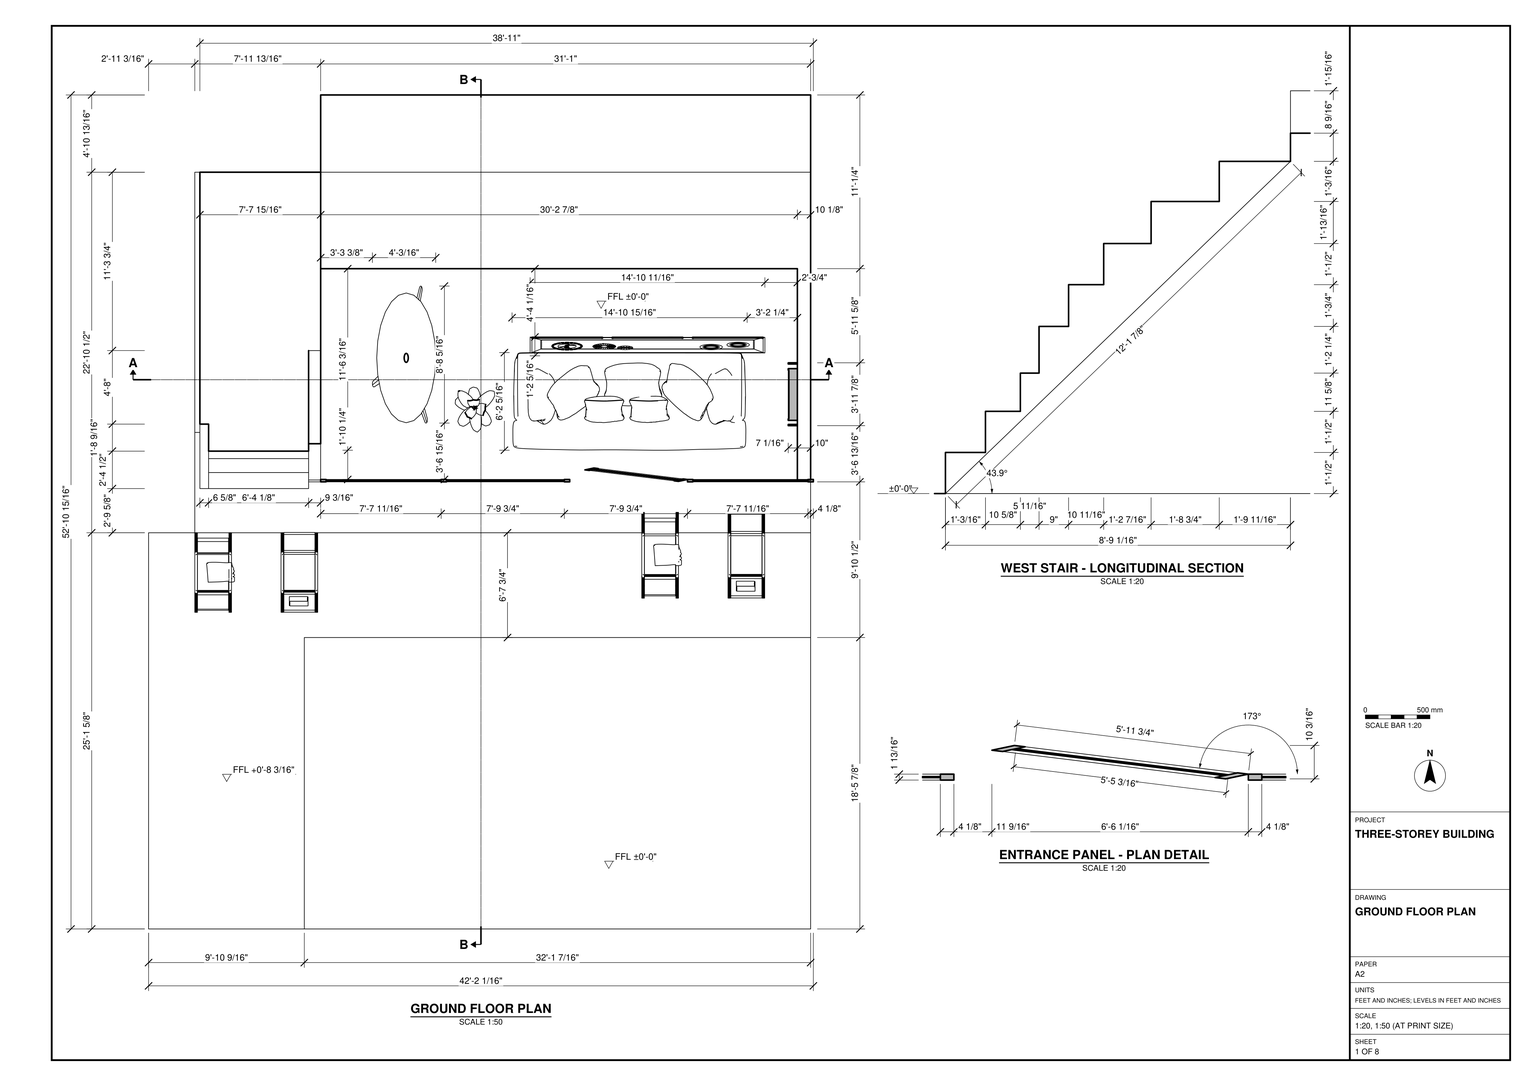
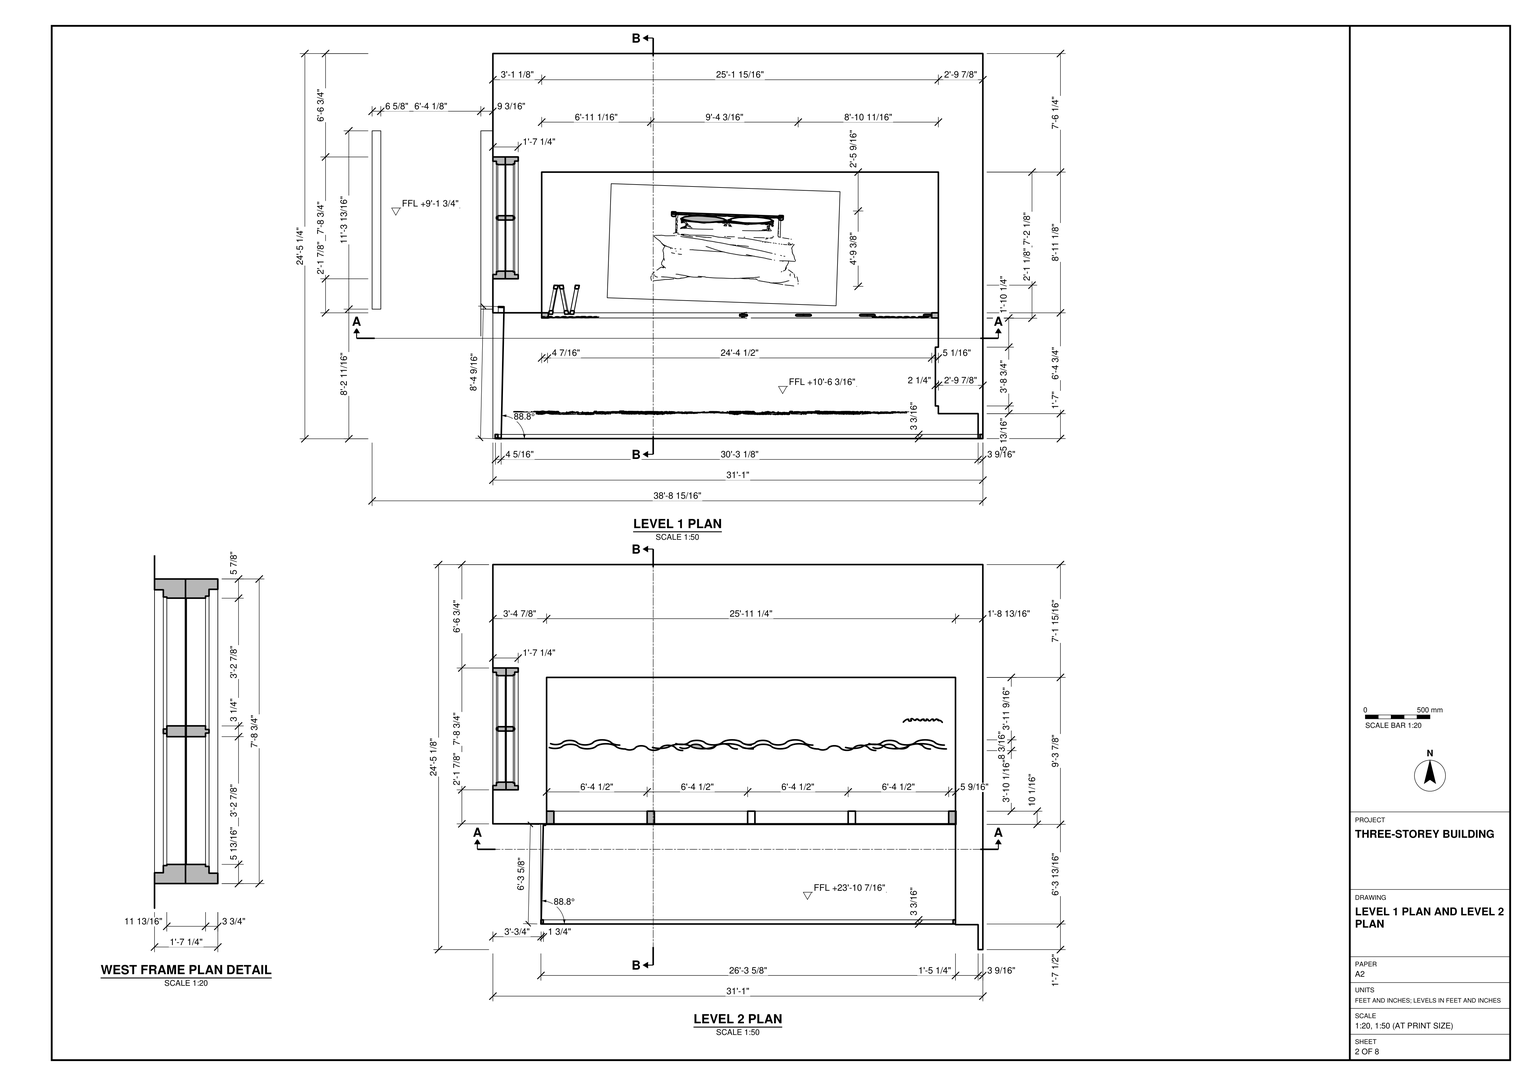
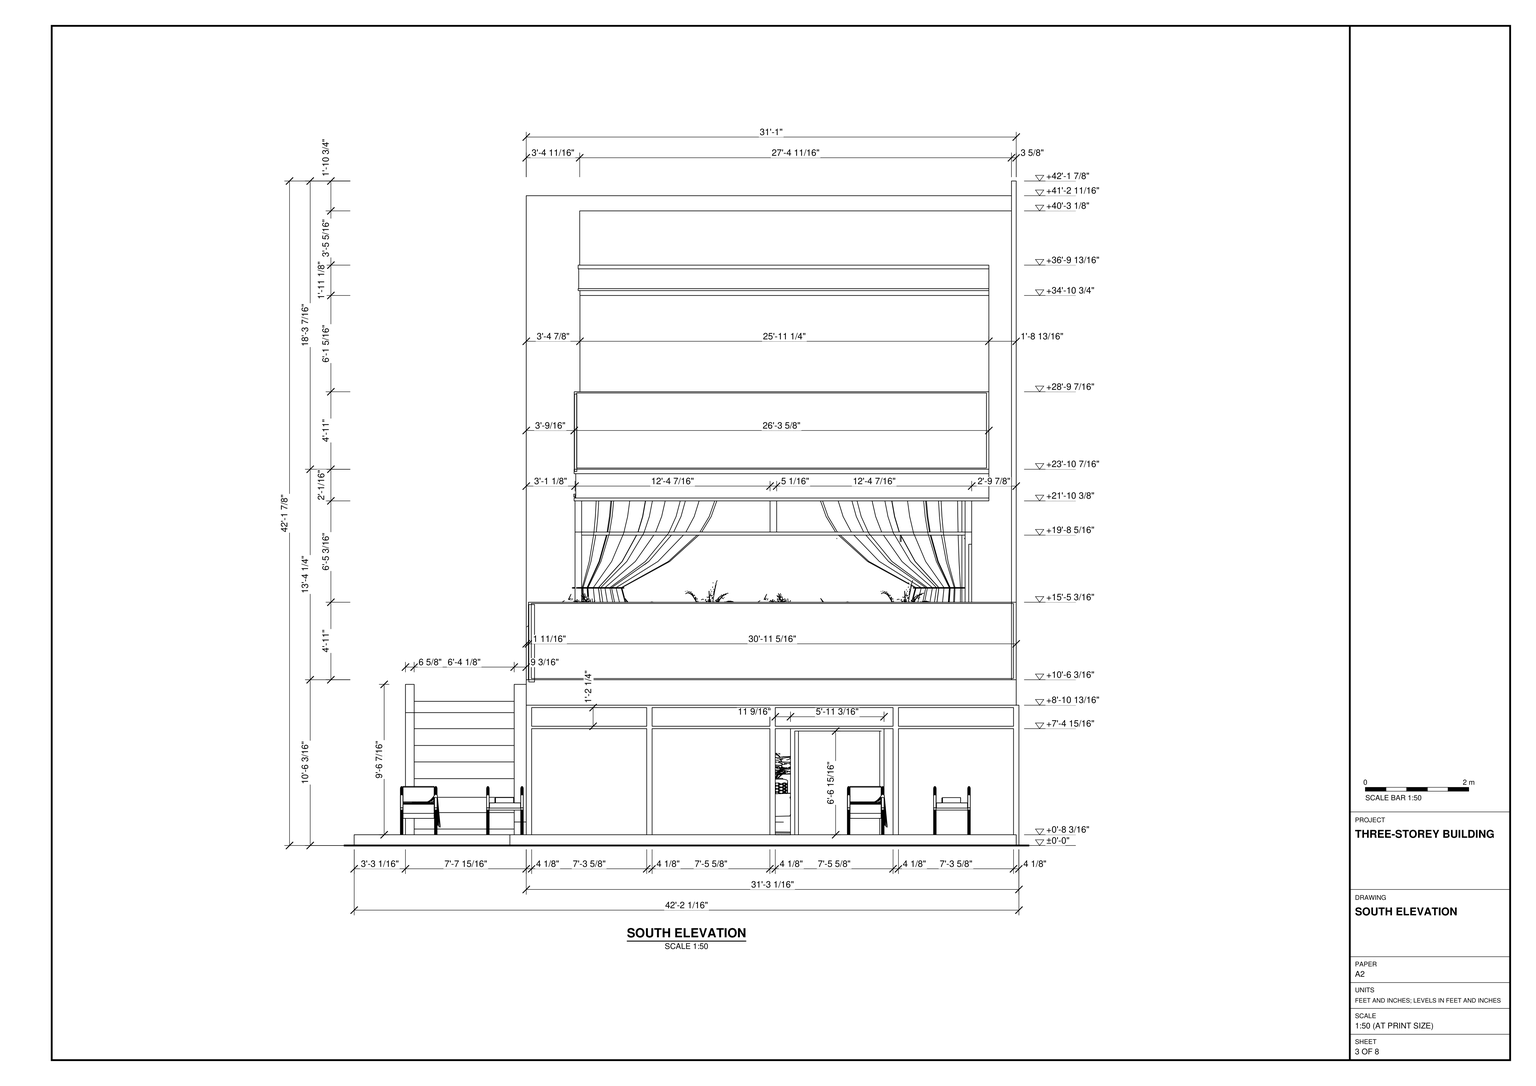
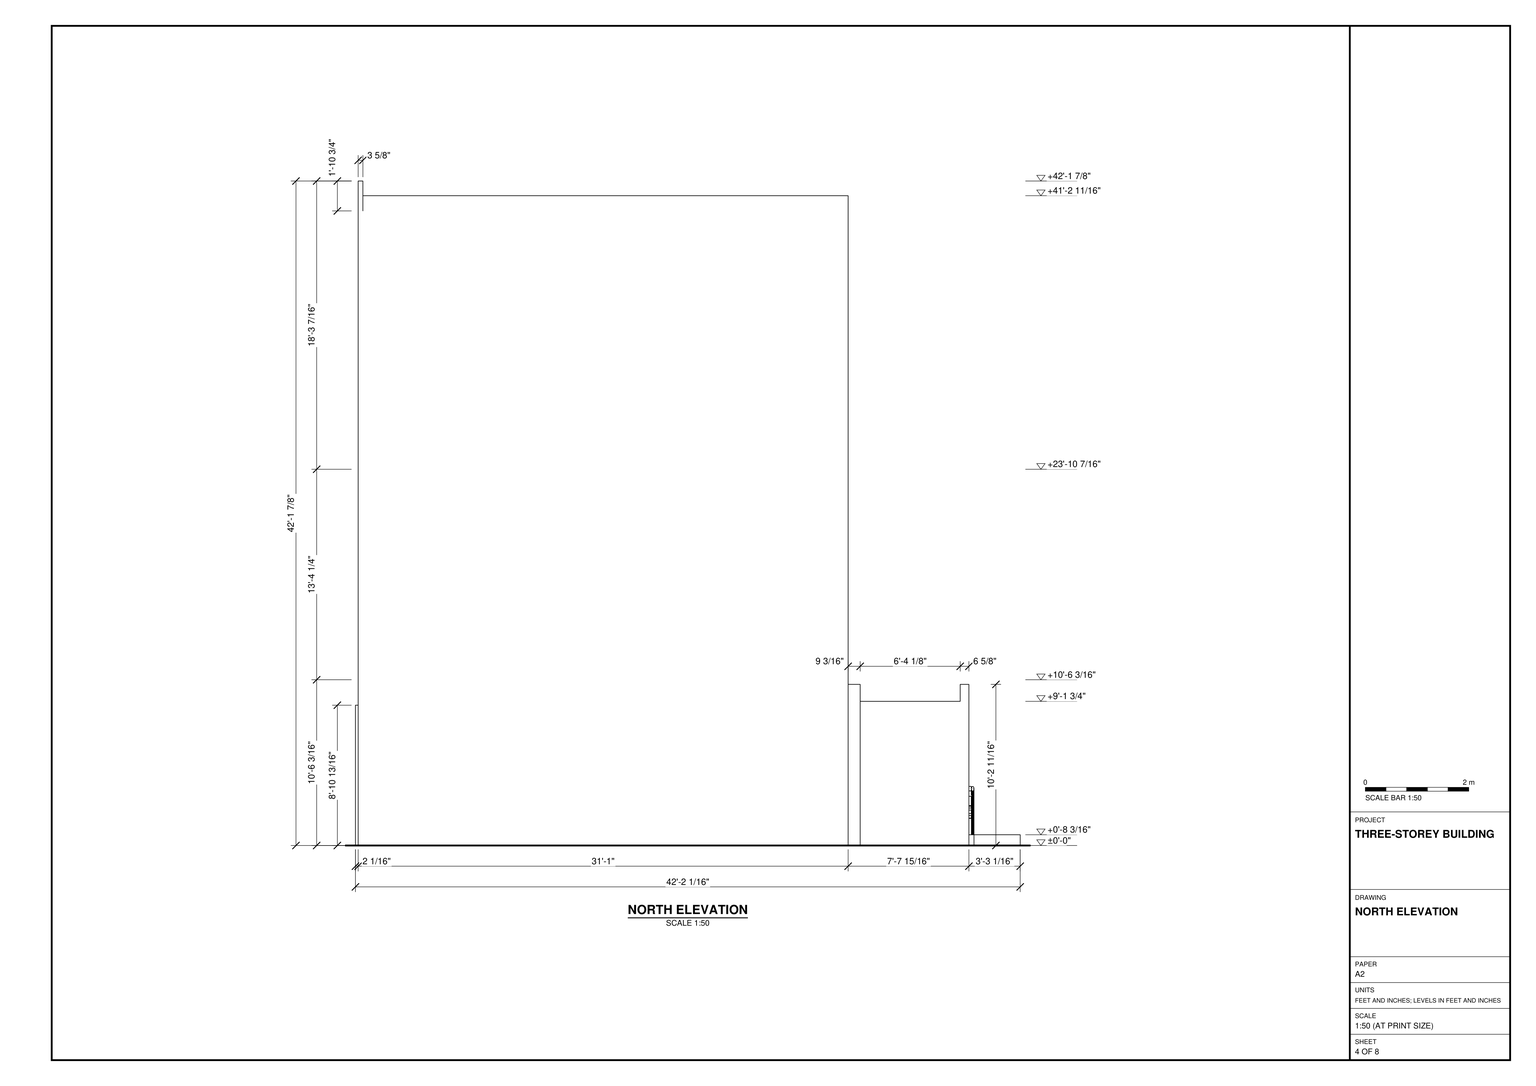
Build the three-storey building and its stepped base in SketchUp from task_files/diagram_01.pdf. Work in feet and inches. Make the overall model 42'-2 1/16" east to west, 52'-10 15/16" north to south and 42'-1 7/8" high. Set the ground floor at ±0'-0", the middle floor at +10'-6 3/16" and the upper floor at +23'-10 7/16".

Use the plans to set out the walls at their drawn thicknesses, the floor slabs, the raised strip beside the forecourt and the exterior stair on the west. Follow the stair section for the treads and landing. At the south entrance, reproduce the framed bays, the panels above them and the angle of the entrance panel. Match the upper floors to the south elevation: the middle balcony spans nearly the full frontage, while the upper balcony is narrower and inset. Include the west window frames, balcony fronts, side walls and roof profile shown on the sheets.

Size and place the ground-floor sofa, the long unit behind it, the oval table and the middle-floor bed from their plan outlines. Place the outdoor seating in the forecourt as drawn. Decor and loose items may be any suitable library components. Keep walls, slabs, roof elements and each furniture or joinery piece in separate groups or components, and use components for repeated parts. Save one SketchUp model as output_files/three_storey_building_with_balconies_and_a_west_stair.skp.

# SketchUp Ruby script. Lengths in inches.
U = 1.inch
M = Sketchup.active_model
def pt(a) = Geom::Point3d.new(a.map { |v| v * U })
def face(e, loops, mat)
  f = e.add_face(loops[0].map { |a| pt(a) })
  loops[1..].each { |l| e.add_face(l.map { |a| pt(a) }).erase! }
  f.material = f.back_material = mat if mat
  f
end
# faces: each face lists its corners as indices into pts; further lists are holes
def faces(e, pts, list, mat = nil) = list.each { |f| face(e, (f[0].is_a?(Array) ? f : [f]).map { |l| l.map { |i| pts[i] } }, mat) }
# xy, xz, yz: faces in a plane at the given z, y or x. An outline is a flat list of corners, or four numbers for a rectangle; further outlines are holes
def ring(l) = l.size == 4 ? [[l[0], l[1]], [l[2], l[1]], [l[2], l[3]], [l[0], l[3]]] : l.each_slice(2).to_a
def flat(e, list, mat, &to3) = list.each { |f| face(e, (f[0].is_a?(Array) ? f : [f]).map { |l| ring(l).map { |u, v| to3.(u, v) } }, mat) }
def xy(e, z, list, mat = nil) = flat(e, list, mat) { |x, y| [x, y, z] }
def xz(e, y, list, mat = nil) = flat(e, list, mat) { |x, z| [x, y, z] }
def yz(e, x, list, mat = nil) = flat(e, list, mat) { |y, z| [x, y, z] }
def lines(e, pts, list) = list.each { |a, b| e.add_line(pt(pts[a]), pt(pts[b])) }
# prism: a flat outline (further loops are holes) pulled along v
def prism(e, loops, v, mat = nil)
  f = face(e, loops, mat); d = Geom::Vector3d.new(v.map { |x| x * U })
  f.pushpull(f.normal.samedirection?(d) ? d.length : -d.length)
end
def box(e, o, s, mat = nil) = prism(e, [[o, [o[0] + s[0], o[1], o[2]], [o[0] + s[0], o[1] + s[1], o[2]], [o[0], o[1] + s[1], o[2]]]], [0, 0, s[2]], mat)
def at(x, y, z, deg = 0) = Geom::Transformation.translation(pt([x, y, z])) * Geom::Transformation.rotation(ORIGIN, Z_AXIS, deg.degrees)
def axes(o, x, y, z) = Geom::Transformation.new([*x, 0, *y, 0, *z, 0, *pt(o).to_a, 1])
def part(name) = M.definitions.add(name)
# library, detail: a bought-in or finely detailed component or shape, given as its bounding box
def library(name, o, s) = part(name).tap { |d| box(d.entities, o, s) }
def detail(e, o, s) = box(e.add_group.entities, o, s)
def put(e, d, t, mat = nil) = e.add_instance(d, t).tap { |i| i.material = mat if mat }
def group(e, t, mat = nil) = e.add_group.tap { |g| g.transformation = t; g.material = mat if mat }.entities
root = M.entities
M.materials.add("123 Glass_Window_WaterBlue").color = [139, 139, 139]
M.materials["123 Glass_Window_WaterBlue"].alpha = 0.1875
M.materials.add("Aluminum Anodized DarkGray").color = [79, 73, 69]
M.materials.add("BeigeGloss_500x700").color = [214, 201, 185]
M.materials.add("Carpet_Frieze_Low").color = [170, 156, 146]
M.materials.add("Carpet_Loop_Low").color = [201, 172, 127]
M.materials["Carpet_Loop_Low"].alpha = 0.3
M.materials.add("Lisanne_Tool_Bag_1").color = [24, 24, 28]
M.materials.add("[Asphalt New]").color = [67, 60, 62]
M.materials.add("[Concrete Form 4x8]").color = [167, 170, 168]
M.materials.add("[Concrete Scored Jointless]").color = [140, 133, 127]
M.materials.add("[Grass Dark Green]").color = [106, 157, 55]
M.materials.add("[Polished Concrete New]").color = [200, 200, 203]
M.materials.add("[Translucent Glass Gray]").color = [128, 128, 128]
M.materials["[Translucent Glass Gray]"].alpha = 0.5
M.materials.add("[Water Sparkling]").color = [45, 182, 216]
M.materials.add("[Wood Floor]").color = [155, 105, 61]
M.materials.add("clear_glass").color = [0, 0, 0]
M.materials["clear_glass"].alpha = 0
M.materials.add("espelho").color = [126, 126, 126]
c1 = library("SOFA\#1",[0.35,-39.08,0.31],[80.46,34.29,30.24])
c2 = library("консоль+и+зеркало",[175.07,156.1,0],[18.49,52.36,84.07])
c3 = library("Group\#82",[0,0,0],[81.1,114.11,11.8125])
c4 = library("floor+lamp",[-134.64,47.3125,-193.76],[13.07,13.16,54.1])
c5 = library("Plant Banana",[3.49,5.74,0],[38.27,39.55,56.51])
c6 = library("glass+door",[90.99,-32.14,0],[118.11,25.15,118.11])
c7 = library("CURTAIN",[20.4,9.88,0],[29.77,2.88,102.36])
c8 = part("Curtain panel")
p = [[17.625,0.0625,78.74],[17.625,0.0625,0],[18.27,0,0],[18.27,0,78.74],[18.92,0.0625,0],[18.92,0.0625,78.74],
  [17,0.25,78.74],[17,0.25,0],[19.55,0.25,0],[19.55,0.25,78.74],[16.43,0.56,78.74],[16.43,0.56,0],
  [20.12,0.56,0],[20.12,0.56,78.74],[6.31,0.6,78.74],[6.31,0.6,0],[6.8125,0.45,0],[6.8125,0.45,78.74],
  [7.33,0.4,0],[7.33,0.4,78.74],[7.86,0.45,0],[7.86,0.45,78.74],[8.36,0.6,0],[8.36,0.6,78.74],
  [5.85,0.85,78.74],[5.85,0.85,0],[8.82,0.85,0],[8.82,0.85,78.74],[15.92,0.97,78.74],[15.92,0.97,0],
  [20.625,0.97,0],[20.625,0.97,78.74],[5.44,1.18,78.74],[5.44,1.18,0],[9.23,1.18,0],[9.23,1.18,78.74],
  [15.51,1.48,78.74],[15.51,1.48,0],[21.04,1.48,0],[21.04,1.48,78.74],[5.11,1.59,78.74],[5.11,1.59,0],
  [9.5625,1.59,0],[9.5625,1.59,78.74],[14.93,2.55,78.74],[14.93,2.55,0],[15.2,2.04,0],[15.2,2.04,78.74],
  [21.34,2.04,0],[21.64,2.59,0],[21.64,2.59,78.74],[21.34,2.04,78.74],[4.63,2.47,78.74],[4.63,2.47,0],
  [4.86,2.04,0],[4.86,2.04,78.74],[9.81,2.04,0],[10.08,2.55,0],[10.08,2.55,78.74],[9.81,2.04,78.74],
  [4.32,2.85,78.74],[4.32,2.85,0],[10.44,2.99,0],[10.44,2.99,78.74],[14.57,2.99,78.74],[14.57,2.99,0],
  [22.03,3.0625,0],[22.03,3.0625,78.74],[0.85,2.85,78.74],[0.85,2.85,0],[1.22,3.15,0],[1.22,3.15,78.74],
  [3.95,3.15,78.74],[3.95,3.15,0],[10.89,3.35,0],[10.89,3.35,78.74],[14.125,3.35,78.74],[14.125,3.35,0],
  [22.5,3.45,0],[22.5,3.45,78.74],[1.65,3.375,0],[1.65,3.375,78.74],[3.53,3.375,78.74],[3.53,3.375,0],
  [2.11,3.52,0],[2.11,3.52,78.74],[3.07,3.52,78.74],[3.07,3.52,0],[11.39,3.625,0],[11.39,3.625,78.74],
  [13.62,3.625,78.74],[13.62,3.625,0],[2.59,3.5625,0],[2.59,3.5625,78.74],[23.04,3.74,0],[23.04,3.74,78.74],
  [11.9375,3.79,0],[11.9375,3.79,78.74],[13.07,3.79,78.74],[13.07,3.79,0],[23.63,3.92,0],[23.63,3.92,78.74],
  [12.51,3.85,0],[12.51,3.85,78.74],[24.25,3.98,0],[24.25,3.98,78.74],[5.51,1.25,0],[5.9,0.93,0],
  [4.95,2.09,0],[5.1875,1.64,0],[6.35,0.69,0],[6.83,0.55,0],[7.33,0.5,0],[7.84,0.55,0],
  [8.32,0.69,0],[8.77,0.93,0],[9.16,1.25,0],[9.48,1.64,0],[9.72,2.09,0],[10,2.61,0],
  [10.375,3.0625,0],[10.83,3.4375,0],[17.64,0.16,0],[18.27,0.1,0],[11.35,3.71,0],[11.92,3.89,0],
  [12.51,3.94,0],[13.09,3.89,0],[20.56,1.04,0],[20.96,1.53,0],[13.66,3.71,0],[14.18,3.4375,0],
  [14.64,3.0625,0],[15.01,2.61,0],[15.29,2.09,0],[15.59,1.53,0],[15.99,1.04,0],[16.48,0.64,0],
  [17.04,0.34,0],[18.9,0.16,0],[19.51,0.34,0],[20.07,0.64,0],[21.26,2.09,0],[21.56,2.64,0],
  [21.96,3.13,0],[22.45,3.53,0],[23,3.83,0],[23.61,4.01,0],[24.24,4.08,0]]
faces(c8.entities,p,[[0,1,2,3],[3,2,4,5],[6,7,1,0],[5,4,8,9],[10,11,7,6],[9,8,12,13],[14,15,16,17],[17,16,18,19],
  [19,18,20,21],[21,20,22,23],[24,25,15,14],[23,22,26,27],[28,29,11,10],[13,12,30,31],[32,33,25,24],[27,26,34,35],
  [36,37,29,28],[31,30,38,39],[40,41,33,32],[35,34,42,43],[44,45,46,37,36,47],[39,38,48,49,50,51],[52,53,54,41,40,55],[43,42,56,57,58,59],
  [60,61,53,52],[58,57,62,63],[64,65,45,44],[50,49,66,67],[68,69,70,71],[72,73,61,60],[63,62,74,75],[76,77,65,64],
  [67,66,78,79],[71,70,80,81],[82,83,73,72],[81,80,84,85],[86,87,83,82],[75,74,88,89],[90,91,77,76],[85,84,92,93],
  [93,92,87,86],[79,78,94,95],[89,88,96,97],[98,99,91,90],[95,94,100,101],[97,96,102,103],[103,102,99,98],[101,100,104,105]])
lines(c8.entities,p,[[106,107],[108,109],[109,106],[107,110],[110,111],[111,112],[112,113],[113,114],[114,115],[115,116],[116,117],[117,118],
  [118,119],[119,120],[120,121],[122,123],[121,124],[124,125],[125,126],[126,127],[128,129],[127,130],[130,131],[131,132],
  [132,133],[133,134],[134,135],[135,136],[136,137],[137,138],[138,122],[123,139],[139,140],[140,141],[141,128],[129,142],
  [142,143],[143,144],[144,145],[145,146],[146,147],[147,148],[148,104]])
c9 = part("Curtain rod section")
yz(c9.entities,0,[[1.55,0.61,1.31,0.64,1.08,0.73,0.88,0.88,0.73,1.08,0.64,1.31,0.61,1.55,0.64,1.79,0.73,2.02,0.88,2.22,1.08,2.37,1.31,2.46,1.55,2.49,1.79,2.46,2.02,2.37,2.22,2.22,2.37,2.02,2.46,1.79,2.49,1.55,2.46,1.31,2.37,1.08,2.22,0.88,2.02,0.73,1.79,0.64]],"espelho")
yz(c9.entities,2.36,[[[1.55,0,1.15,0.05,0.78,0.21,0.45,0.45,0.21,0.78,0.05,1.15,0,1.55,0.05,1.95,0.21,2.33,0.45,2.65,0.78,2.89,1.15,3.05,1.55,3.1,1.95,3.05,2.33,2.89,2.65,2.65,2.89,2.33,3.05,1.95,3.1,1.55,3.05,1.15,2.89,0.78,2.65,0.45,2.33,0.21,1.95,0.05],[1.55,0.61,1.79,0.64,2.02,0.73,2.22,0.88,2.37,1.08,2.46,1.31,2.49,1.55,2.46,1.79,2.37,2.02,2.22,2.22,2.02,2.37,1.79,2.46,1.55,2.49,1.31,2.46,1.08,2.37,0.88,2.22,0.73,2.02,0.64,1.79,0.61,1.55,0.64,1.31,0.73,1.08,0.88,0.88,1.08,0.73,1.31,0.64]]],"espelho")
yz(c9.entities,3.15,[[[1.55,0,1.95,0.05,2.33,0.21,2.65,0.45,2.89,0.78,3.05,1.15,3.1,1.55,3.05,1.95,2.89,2.33,2.65,2.65,2.33,2.89,1.95,3.05,1.55,3.1,1.15,3.05,0.78,2.89,0.45,2.65,0.21,2.33,0.05,1.95,0,1.55,0.05,1.15,0.21,0.78,0.45,0.45,0.78,0.21,1.15,0.05],[1.55,0.61,1.31,0.64,1.08,0.73,0.88,0.88,0.73,1.08,0.64,1.31,0.61,1.55,0.64,1.79,0.73,2.02,0.88,2.22,1.08,2.37,1.31,2.46,1.55,2.49,1.79,2.46,2.02,2.37,2.22,2.22,2.37,2.02,2.46,1.79,2.49,1.55,2.46,1.31,2.37,1.08,2.22,0.88,2.02,0.73,1.79,0.64]]],"espelho")
yz(c9.entities,61.24,[[1.55,0.61,1.79,0.64,2.02,0.73,2.22,0.88,2.37,1.08,2.46,1.31,2.49,1.55,2.46,1.79,2.37,2.02,2.22,2.22,2.02,2.37,1.79,2.46,1.55,2.49,1.31,2.46,1.08,2.37,0.88,2.22,0.73,2.02,0.64,1.79,0.61,1.55,0.64,1.31,0.73,1.08,0.88,0.88,1.08,0.73,1.31,0.64]],"espelho")
p = [[2.36,1.15,0.05],[2.36,1.55,0],[3.15,1.55,0],[3.15,1.15,0.05],[2.36,1.95,0.05],[3.15,1.95,0.05],
  [2.36,0.78,0.21],[3.15,0.78,0.21],[2.36,2.33,0.21],[3.15,2.33,0.21],[2.36,0.45,0.45],[3.15,0.45,0.45],
  [2.36,2.65,0.45],[3.15,2.65,0.45],[2.36,0.21,0.78],[3.15,0.21,0.78],[2.36,2.89,0.78],[3.15,2.89,0.78],
  [2.36,1.31,0.64],[2.36,1.08,0.73],[0,1.08,0.73],[0,1.31,0.64],[3.15,1.31,0.64],[3.15,1.08,0.73],
  [61.24,1.31,0.64],[61.24,1.08,0.73],[2.36,1.55,0.61],[0,1.55,0.61],[3.15,1.55,0.61],[61.24,1.55,0.61],
  [2.36,1.79,0.64],[0,1.79,0.64],[3.15,1.79,0.64],[61.24,1.79,0.64],[2.36,2.02,0.73],[0,2.02,0.73],
  [3.15,2.02,0.73],[61.24,2.02,0.73],[2.36,0.88,0.88],[0,0.88,0.88],[3.15,0.88,0.88],[61.24,0.88,0.88],
  [2.36,2.22,0.88],[0,2.22,0.88],[3.15,2.22,0.88],[61.24,2.22,0.88],[2.36,0.05,1.15],[3.15,0.05,1.15],
  [2.36,3.05,1.15],[3.15,3.05,1.15],[2.36,0.73,1.08],[0,0.73,1.08],[3.15,0.73,1.08],[61.24,0.73,1.08],
  [2.36,2.37,1.08],[0,2.37,1.08],[3.15,2.37,1.08],[61.24,2.37,1.08],[2.36,0,1.55],[3.15,0,1.55],
  [2.36,0.64,1.31],[0,0.64,1.31],[3.15,0.64,1.31],[61.24,0.64,1.31],[2.36,2.46,1.31],[0,2.46,1.31],
  [3.15,2.46,1.31],[61.24,2.46,1.31],[2.36,3.1,1.55],[3.15,3.1,1.55],[2.36,0.61,1.55],[0,0.61,1.55],
  [3.15,0.61,1.55],[61.24,0.61,1.55],[2.36,2.49,1.55],[0,2.49,1.55],[3.15,2.49,1.55],[61.24,2.49,1.55],
  [2.36,0.05,1.95],[3.15,0.05,1.95],[2.36,0.64,1.79],[0,0.64,1.79],[3.15,0.64,1.79],[61.24,0.64,1.79],
  [2.36,2.46,1.79],[0,2.46,1.79],[3.15,2.46,1.79],[61.24,2.46,1.79],[2.36,3.05,1.95],[3.15,3.05,1.95],
  [2.36,0.73,2.02],[0,0.73,2.02],[3.15,0.73,2.02],[61.24,0.73,2.02],[2.36,2.37,2.02],[0,2.37,2.02],
  [3.15,2.37,2.02],[61.24,2.37,2.02],[2.36,0.21,2.33],[3.15,0.21,2.33],[2.36,0.88,2.22],[0,0.88,2.22],
  [3.15,0.88,2.22],[61.24,0.88,2.22],[2.36,2.22,2.22],[0,2.22,2.22],[3.15,2.22,2.22],[61.24,2.22,2.22],
  [2.36,2.89,2.33],[3.15,2.89,2.33],[2.36,1.08,2.37],[0,1.08,2.37],[3.15,1.08,2.37],[61.24,1.08,2.37],
  [2.36,2.02,2.37],[0,2.02,2.37],[3.15,2.02,2.37],[61.24,2.02,2.37],[2.36,0.45,2.65],[3.15,0.45,2.65],
  [2.36,2.65,2.65],[3.15,2.65,2.65],[2.36,1.31,2.46],[0,1.31,2.46],[3.15,1.31,2.46],[61.24,1.31,2.46],
  [2.36,1.79,2.46],[0,1.79,2.46],[3.15,1.79,2.46],[61.24,1.79,2.46],[2.36,1.55,2.49],[0,1.55,2.49],
  [3.15,1.55,2.49],[61.24,1.55,2.49],[2.36,0.78,2.89],[3.15,0.78,2.89],[2.36,2.33,2.89],[3.15,2.33,2.89],
  [2.36,1.15,3.05],[3.15,1.15,3.05],[2.36,1.95,3.05],[3.15,1.95,3.05],[2.36,1.55,3.1],[3.15,1.55,3.1]]
faces(c9.entities,p,[[0,1,2,3],[1,4,5,2],[6,0,3,7],[4,8,9,5],[10,6,7,11],[8,12,13,9],[14,10,11,15],[12,16,17,13],
  [18,19,20,21],[19,18,22,23],[24,25,23,22],[26,18,21,27],[18,26,28,22],[29,24,22,28],[30,26,27,31],[26,30,32,28],
  [33,29,28,32],[34,30,31,35],[30,34,36,32],[37,33,32,36],[19,38,39,20],[38,19,23,40],[25,41,40,23],[42,34,35,43],
  [34,42,44,36],[45,37,36,44],[46,14,15,47],[16,48,49,17],[38,50,51,39],[50,38,40,52],[41,53,52,40],[54,42,43,55],
  [42,54,56,44],[57,45,44,56],[58,46,47,59],[50,60,61,51],[60,50,52,62],[53,63,62,52],[64,54,55,65],[54,64,66,56],
  [67,57,56,66],[48,68,69,49],[60,70,71,61],[70,60,62,72],[63,73,72,62],[74,64,65,75],[64,74,76,66],[77,67,66,76],
  [78,58,59,79],[70,80,81,71],[80,70,72,82],[73,83,82,72],[84,74,75,85],[74,84,86,76],[87,77,76,86],[68,88,89,69],
  [80,90,91,81],[90,80,82,92],[83,93,92,82],[94,84,85,95],[84,94,96,86],[97,87,86,96],[98,78,79,99],[90,100,101,91],
  [100,90,92,102],[93,103,102,92],[104,94,95,105],[94,104,106,96],[107,97,96,106],[88,108,109,89],[100,110,111,101],[110,100,102,112],
  [103,113,112,102],[114,104,105,115],[104,114,116,106],[117,107,106,116],[118,98,99,119],[108,120,121,109],[110,122,123,111],[122,110,112,124],
  [113,125,124,112],[126,114,115,127],[114,126,128,116],[129,117,116,128],[122,130,131,123],[130,122,124,132],[125,133,132,124],[130,126,127,131],
  [126,130,132,128],[133,129,128,132],[134,118,119,135],[120,136,137,121],[138,134,135,139],[136,140,141,137],[142,138,139,143],[140,142,143,141]],"espelho")
c10 = part("Curtain rod")
put(c10.entities,c9,axes([3.125,-0.76,-71.54],[0,0,1.25313],[0,1.25313,0],[-1.25313,0,0]))
put(c10.entities,c9,axes([3.125,3.125,81],[0,0,-1.25313],[0,-1.25313,0],[-1.25313,0,0]))
c11 = part("Group\#25")
put(c11.entities,c8,axes([-0.76,0,0],[0.8979,0,0],[0,1,0],[0,0,1]),"Carpet_Frieze_Low")
put(c11.entities,c8,axes([37.23,0,0],[0.9782,0,0],[0,1,0],[0,0,1]),"Carpet_Frieze_Low")
c12 = part("curtain2")
p = [[59.99,12.8,78.74],[59.99,12.8,-38.1875],[60.15,12.52,-38.1875],[60.15,12.52,78.74],[66.72,13.7,-38.1875],[66.72,13.7,78.74],
  [73.91,13.97,78.74],[73.91,13.97,-38.1875],[49.31,14.13,-38.1875],[49.31,14.13,78.74],[2.67,12.52,-38.1875],[2.67,12.52,78.74],
  [-8.17,14.13,-38.1875],[-8.17,14.13,78.74],[2.51,12.8,78.74],[2.51,12.8,-38.1875],[16.42,13.97,78.74],[16.42,13.97,-38.1875],
  [9.24,13.7,-38.1875],[9.24,13.7,78.74]]
lines(c12.entities,p,[[0,1],[2,3],[4,5],[6,7],[8,9],[10,11],[12,13],[14,15],[16,17],[18,19]])
put(c12.entities,c8,axes([64.94,10.15,-38.1875],[0.73,0,0],[0,1,0],[0,0,1.485]),"Carpet_Loop_Low")
put(c12.entities,c8,axes([48.6875,11.28,-38.1875],[0.73,0,0],[0,1,0],[0,0,1.485]),"Carpet_Loop_Low")
put(c12.entities,c8,axes([25.83,10.15,-38.1875],[0.96815,0,0],[0,1,0],[0,0,1.485]),"Carpet_Loop_Low")
put(c12.entities,c8,axes([56.28,10.09,-38.1875],[1.28298,0,0],[0,1,0],[0,0,1.485]),"Carpet_Loop_Low")
put(c12.entities,c10,axes([25.47,12.88,78.42],[0,0,-0.798],[0,0.798,0],[0.798,0,0]))
put(c12.entities,c8,axes([7.46,10.15,-38.1875],[0.73,0,0],[0,1,0],[0,0,1.485]),"Carpet_Loop_Low")
put(c12.entities,c8,axes([-1.2,10.09,-38.1875],[1.28298,0,0],[0,1,0],[0,0,1.485]),"Carpet_Loop_Low")
put(c12.entities,c8,axes([-8.79,11.28,-38.1875],[0.73,0,0],[0,1,0],[0,0,1.485]),"Carpet_Loop_Low")
put(c12.entities,c8,axes([-31.65,10.15,-38.1875],[0.96815,0,0],[0,1,0],[0,0,1.485]),"Carpet_Loop_Low")
put(c12.entities,c11,axes([27.05,7.18,-38.1875],[0.98,0,0],[0,1,0],[0,0,1.485]))
put(c12.entities,c11,axes([-30.43,7.18,-38.1875],[0.98,0,0],[0,1,0],[0,0,1.485]))
c13 = part("Curtains")
put(c13.entities,c12,axes([31.62,15.375,38.1875],[1,0,0],[0,-1,0],[0,0,1]))
c14 = part("Window frame member")
box(c14.entities,[0,0,3.9375],[3.9375,9.65,110.23])
c15 = part("Window frame member \#1")
box(c15.entities,[0,0,-101.16],[3.9375,9.65,221.03])
c16 = library("Greenwindows Roller Blinds Q System\#14",[-2.45,-186.1875,144.74],[68.81,2.71,70.55])
c17 = part("Window+Glass+01")
put(c17.entities,c14,at(0,3.9375,0,-89.986),"Aluminum Anodized DarkGray")
put(c17.entities,c15,axes([0,119.87,3.9375],[0,0,-1],[1,0,0],[0,-1,0]),"Aluminum Anodized DarkGray")
put(c17.entities,c14,at(0,58.21,0,-89.986),"Aluminum Anodized DarkGray")
put(c17.entities,c15,axes([0,119.87,118.11],[0,0,-1],[1,0,0],[0,-1,0]),"Aluminum Anodized DarkGray")
put(c17.entities,c16,axes([-125.93,60.17,-42.69],[0.00063,0.73001,0],[-0.72848,0.00063,0],[0,0,0.72864]))
put(c17.entities,c16,axes([-125.93,114.44,-42.69],[0.00063,0.73001,0],[-0.72848,0.00063,0],[0,0,0.72864]))
put(c17.entities,c16,axes([-125.93,5.9,-42.69],[0.00063,0.73001,0],[-0.72848,0.00063,0],[0,0,0.72864]))
put(c17.entities,c16,axes([-125.93,168.71,-42.69],[0.00063,0.73001,0],[-0.72848,0.00063,0],[0,0,0.72864]))
put(c17.entities,c14,at(0,112.48,0,-89.986),"Aluminum Anodized DarkGray")
put(c17.entities,c14,at(0,166.75,0,-89.986),"Aluminum Anodized DarkGray")
put(c17.entities,c14,at(0,221.02,0,-89.986),"Aluminum Anodized DarkGray")
g1 = group(c17.entities,at(-0.42,-51.41,0))
prism(g1,[[[0.41,272.4375,0],[0.4,51.42,0],[0,51.42,0],[0.01,272.4375,0]]],[0,0,118.11],"123 Glass_Window_WaterBlue")
c18 = part("window full")
xy(c18.entities,0,[[0,0,14.17,66.54]])
xy(c18.entities,2.26,[[12.2,2.26,14.17,64.28]],"[Wood Floor]")
xy(c18.entities,2.36,[[0,2.36,1.97,64.17]],"[Wood Floor]")
xy(c18.entities,3.74,[[11.42,3.74,12.2,32.875],[11.42,33.66,12.2,62.79]],"[Wood Floor]")
xy(c18.entities,3.9375,[[1.97,3.9375,2.76,32.77],[1.97,33.76,2.76,62.6]],"[Wood Floor]")
xy(c18.entities,4.18,[[2.76,4.18,7.09,32.09],[7.09,4.18,11.42,32.09],[2.76,34.45,7.09,62.35],[7.09,34.45,11.42,62.35]],"[Wood Floor]")
xy(c18.entities,69.83,[[2.76,4.18,7.09,32.09],[7.09,32.09,11.42,34.45],[2.76,34.45,7.09,62.35]])
xy(c18.entities,69.83,[[7.09,4.18,11.42,32.09],[7.09,34.45,11.42,62.35]],"[Wood Floor]")
xy(c18.entities,70.08,[[1.97,3.9375,2.76,32.77],[1.97,33.76,2.76,62.6]])
xy(c18.entities,70.27,[[11.42,32.875,12.2,33.66]])
xy(c18.entities,70.27,[[11.42,3.74,12.2,32.875],[11.42,33.66,12.2,62.79]],"[Wood Floor]")
xy(c18.entities,71.65,[[0,2.36,1.97,64.17]])
xy(c18.entities,71.76,[[12.2,2.26,14.17,64.28]],"[Wood Floor]")
xy(c18.entities,74.02,[[0,0,14.17,66.54]],"[Wood Floor]")
xz(c18.entities,0,[[0,0,14.17,74.02]],"[Wood Floor]")
xz(c18.entities,2.26,[[12.2,2.26,14.17,71.76]],"[Wood Floor]")
xz(c18.entities,2.36,[[0,2.36,1.97,71.65]],"[Wood Floor]")
xz(c18.entities,3.74,[[11.42,3.74,12.2,70.27]],"[Wood Floor]")
xz(c18.entities,3.9375,[[1.97,3.9375,2.76,70.08]],"[Wood Floor]")
xz(c18.entities,4.18,[[2.76,4.18,7.09,69.83],[7.09,4.18,11.42,69.83]],"[Wood Floor]")
xz(c18.entities,32.09,[[2.76,4.18,11.42,69.83]],"[Wood Floor]")
xz(c18.entities,32.77,[[1.97,3.9375,2.76,70.08]],"[Wood Floor]")
xz(c18.entities,32.875,[[11.42,3.74,12.2,70.27]],"[Wood Floor]")
xz(c18.entities,33.66,[[11.42,3.74,12.2,47.88],[11.42,47.88,12.2,70.27]],"[Wood Floor]")
xz(c18.entities,33.76,[[1.97,3.9375,2.76,70.08]],"[Wood Floor]")
xz(c18.entities,34.45,[[2.76,4.18,11.42,69.83]],"[Wood Floor]")
xz(c18.entities,62.35,[[2.76,4.18,7.09,69.83],[7.09,4.18,11.42,69.83]],"[Wood Floor]")
xz(c18.entities,62.6,[[1.97,3.9375,2.76,70.08]],"[Wood Floor]")
xz(c18.entities,62.79,[[11.42,3.74,12.2,70.27]],"[Wood Floor]")
xz(c18.entities,64.17,[[0,2.36,1.97,71.65]],"[Wood Floor]")
xz(c18.entities,64.28,[[12.2,2.26,14.17,71.76]],"[Wood Floor]")
xz(c18.entities,66.54,[[0,0,14.17,74.02]],"[Wood Floor]")
yz(c18.entities,0,[[[0,0,66.54,74.02],[2.36,2.36,64.17,71.65]]],"[Wood Floor]")
yz(c18.entities,1.97,[[[2.36,2.36,64.17,71.65],[33.76,3.9375,62.6,70.08],[3.9375,3.9375,32.77,70.08]]],"[Wood Floor]")
yz(c18.entities,2.76,[[32.77,3.9375,33.76,4.18],[32.77,4.18,33.76,69.83],[32.77,69.83,33.76,70.08]])
yz(c18.entities,2.76,[[[3.9375,3.9375,32.77,70.08],[4.18,4.18,32.09,69.83]],[[33.76,3.9375,62.6,70.08],[34.45,4.18,62.35,69.83]]],"[Wood Floor]")
yz(c18.entities,7.09,[[4.18,4.18,62.35,69.83]],"[Translucent Glass Gray]")
yz(c18.entities,11.42,[[32.875,69.83,33.66,70.27]])
yz(c18.entities,11.42,[[[3.74,3.74,32.875,70.27],[4.18,4.18,32.09,69.83]],[[33.66,3.74,62.79,70.27],[34.45,4.18,62.35,69.83]]],"[Wood Floor]")
yz(c18.entities,12.2,[[[2.26,2.26,64.28,71.76],[3.74,3.74,32.875,70.27],[33.66,3.74,62.79,70.27]]],"[Wood Floor]")
yz(c18.entities,14.17,[[[0,0,66.54,74.02],[2.26,2.26,64.28,71.76]]],"[Wood Floor]")
p = [[11.42,32.875,70.27],[11.42,32.875,70.28]]
lines(c18.entities,p,[[0,1]])
c19 = library("Curtains (1)",[0,0,0],[101.19,6.19,107.53])
c20 = library("girl bed",[-23.97,-20.87,3.43],[151.58,123.63,59.53])
c21 = library("36",[-44.7,-74.43,-0.38],[89.21,170.96,60.16])
c22 = part("Group\#27")
g2 = group(c22.entities,at(0,0,0))
xy(g2,0,[[0,4.33,1184.25,7.93]],"BeigeGloss_500x700")
xy(g2,8.5,[[6.89,4.33,1177.36,7.93]],"BeigeGloss_500x700")
xy(g2,539.53,[[6.89,4.33,1177.36,7.93]],"BeigeGloss_500x700")
xy(g2,548.03,[[0,4.33,1184.25,7.93]],"BeigeGloss_500x700")
xz(g2,4.33,[[[0,0,1184.25,548.03],[6.89,8.5,1177.36,539.53]]],"BeigeGloss_500x700")
xz(g2,7.93,[[6.89,8.5,1177.36,539.53]])
xz(g2,7.93,[[[0,0,1184.25,548.03],[6.89,8.5,1177.36,539.53]]],"BeigeGloss_500x700")
yz(g2,0,[[4.33,0,7.93,548.03]],"BeigeGloss_500x700")
yz(g2,6.89,[[4.33,8.5,7.93,539.53]],"BeigeGloss_500x700")
yz(g2,1177.36,[[4.33,8.5,7.93,539.53]],"BeigeGloss_500x700")
yz(g2,1184.25,[[4.33,0,7.93,548.03]],"BeigeGloss_500x700")
c23 = library("Group\#135",[0,0,0],[78.99,27.95,36.77])
c24 = library("Group\#137",[0,0,0],[78.76,30.32,37.61])
xy(root,0,[[35.1875,301.625,504,301.625,504,341.8,493.9,341.8,493.9,502.68,131.01,502.68,131.01,340.4,121.83,340.4,121.83,335.27,39.07,335.27,39.07,378.02,35.1875,378.02],[121.83,340.4,131.01,440.33],[493.9,341.8,504,341.8,504,576.125,131.01,576.125,131.01,502.68,493.9,502.68],[35.1875,378.02,39.07,576.125],[131.01,576.125,504,634.9375]])
xy(root,0,[[118.5625,0,504,221.875]],"[Water Sparkling]")
xy(root,8.1875,[[0,0,118.5625,0,118.5625,221.875,504,221.875,504,301.625,0,301.625]],"[Polished Concrete New]")
xy(root,12.52,[[45.69,335.27,121.83,347.46]])
xy(root,17.89,[[121.83,340.4,131.01,341.8]])
xy(root,25.04,[[45.69,347.46,121.83,358.08]])
xy(root,36.68,[[45.69,358.08,121.83,363.77]])
xy(root,50.9,[[45.69,363.77,121.83,372.77]])
xy(root,63.62,[[45.69,372.77,121.83,383.46]])
xy(root,76.14,[[45.69,383.46,121.83,397.9]])
xy(root,88.95,[[45.69,397.9,121.83,418.65]])
xy(root,101.16,[[45.69,418.65,121.83,440.33]])
xy(root,106.8125,[[131.01,341.8,493.9,502.68]])
xy(root,109.75,[[45.69,440.33,121.83,576.125]])
xy(root,122.66,[[39.07,440.33,45.69,576.125],[121.83,440.33,131.01,576.125],[131.01,463.45,140.45,556.2]])
xy(root,126.1875,[[131.01,341.8,500.4,341.8,500.4,360.8,470.12,360.8,470.12,366.64,467.87,366.64,467.87,411.39,470.12,411.39,470.12,544.68,168.15,544.68,168.15,437.55,131.01,437.55]])
xy(root,229.35,[[467.87,366.64,470.12,411.39]],"[Grass Dark Green]")
xy(root,238.01,[[131.01,463.45,140.45,556.2]])
xy(root,262.36,[[470.12,360.8,483.18,361.05],[167.46,361.05,167.46,437.55,168.15,437.55,168.15,544.68,470.12,544.68,470.12,361.05]])
xy(root,264.55,[[167.46,361.05,483.18,362.3],[167.46,362.3,168.71,437.55]])
xy(root,283.07,[[167.46,361.3,483.18,362.3],[167.46,362.3,168.71,437.55]])
xy(root,286.4375,[[167.46,361.3,483.18,361.3,483.18,549.02,171.9,549.02,171.9,437.55,167.46,437.55]])
xy(root,295.33,[[131.01,463.45,141.01,556.2]])
xy(root,385.11,[[171.9,482.46,483.18,549.02]])
xy(root,391.35,[[131.01,463.45,141.01,556.2]])
xy(root,413.49,[[131.01,566.8,157.89,615.11]])
xy(root,422.44,[[170.52,362.3,170.52,437.55,171.9,437.55,171.9,482.46,483.18,482.46,483.18,362.3]],"[Wood Floor]")
xy(root,423.93,[[170.96,361.3,483.18,362.3],[170.52,362.3,170.96,437.55]])
xy(root,439.01,[[170.52,359.49,170.96,437.55],[170.96,359.49,483.18,361.3]])
xy(root,441.82,[[170.52,359.49,483.18,360.8],[170.52,360.8,171.71,437.55]])
xy(root,475.36,[[131.01,566.8,157.89,615.11]])
xy(root,483.125,[[171.71,360.8,500.4,437.55]])
xy(root,494.6875,[[131.01,437.55,500.4,634.9375]])
xy(root,505.875,[[500.4,341.8,504,634.9375]])
xz(root,0,[[0,0,118.5625,8.1875]])
xz(root,221.875,[[118.5625,0,504,8.1875]])
xz(root,301.625,[[0,0,35.1875,8.1875],[35.1875,0,504,8.1875]])
xz(root,335.27,[[45.69,0,121.83,12.52]])
xz(root,340.4,[[121.83,0,131.01,17.89]])
xz(root,341.8,[[493.9,0,504,0,504,126.1875,131.01,126.1875,131.01,106.8125,493.9,106.8125]])
xz(root,341.8,[[500.4,126.1875,504,505.875]],"[Concrete Scored Jointless]")
xz(root,347.46,[[45.69,12.52,121.83,25.04]])
xz(root,358.08,[[45.69,25.04,121.83,36.68]])
xz(root,359.49,[[170.52,439.01,483.18,441.82]],"[Asphalt New]")
xz(root,360.8,[[470.12,126.1875,500.4,126.1875,500.4,483.125,171.71,483.125,171.71,441.82,483.18,441.82,483.18,262.36,470.12,262.36]])
xz(root,361.05,[[167.46,262.36,483.18,264.55]],"[Asphalt New]")
xz(root,361.3,[[167.46,283.07,483.18,286.4375]],"[Asphalt New]")
xz(root,361.3,[[170.96,423.93,483.18,439.01]],"[Concrete Scored Jointless]")
xz(root,362.3,[[170.52,422.44,483.18,423.93]],"[Asphalt New]")
xz(root,362.3,[[168.71,264.55,483.18,283.07]],"[Concrete Scored Jointless]")
xz(root,363.77,[[45.69,36.68,121.83,50.9]])
xz(root,366.64,[[467.87,126.1875,470.12,229.35]],"[Grass Dark Green]")
xz(root,372.77,[[45.69,50.9,121.83,63.62]])
xz(root,383.46,[[45.69,63.62,121.83,76.14]])
xz(root,397.9,[[45.69,76.14,121.83,88.95]])
xz(root,411.39,[[467.87,126.1875,470.12,229.35]],"[Grass Dark Green]")
xz(root,418.65,[[45.69,88.95,121.83,101.16]])
xz(root,437.55,[[131.01,126.1875,168.15,126.1875,168.15,262.36,167.46,262.36,167.46,264.55,168.71,264.55,168.71,283.07,167.46,283.07,167.46,286.4375,171.9,286.4375,171.9,422.44,170.52,422.44,170.52,423.93,170.96,423.93,170.96,439.01,170.52,439.01,170.52,441.82,171.71,441.82,171.71,483.125,500.4,483.125,500.4,494.6875,131.01,494.6875]])
xz(root,440.33,[[39.07,101.16,45.69,122.66],[45.69,101.16,121.83,109.75]])
xz(root,463.45,[[131.01,122.66,140.45,238.01],[131.01,295.33,141.01,391.35]])
xz(root,482.46,[[171.9,385.11,483.18,422.44]],"[Concrete Scored Jointless]")
xz(root,502.68,[[131.01,0,493.9,106.8125]])
xz(root,544.68,[[168.15,126.1875,470.12,262.36]])
xz(root,549.02,[[171.9,286.4375,483.18,385.11]])
xz(root,556.2,[[131.01,122.66,140.45,238.01],[131.01,295.33,141.01,391.35]])
xz(root,566.8,[[131.01,413.49,157.89,475.36]])
xz(root,576.125,[[39.07,0,39.07,122.66,45.69,122.66,45.69,109.75,121.83,109.75,121.83,0],[121.83,0,131.01,122.66]])
xz(root,615.11,[[131.01,413.49,157.89,475.36]])
xz(root,634.9375,[[131.01,0,131.01,494.6875,500.4,494.6875,500.4,505.875,504,505.875,504,0]])
yz(root,0,[[0,0,301.625,8.1875]],"[Concrete Form 4x8]")
yz(root,39.07,[[335.27,0,440.33,101.16,440.33,122.66,576.125,122.66,576.125,0]])
yz(root,45.69,[[335.27,0,335.27,12.52,347.46,12.52,347.46,25.04,358.08,25.04,358.08,36.68,363.77,36.68,363.77,50.9,372.77,50.9,372.77,63.62,383.46,63.62,383.46,76.14,397.9,76.14,397.9,88.95,418.65,88.95,418.65,101.16,440.33,101.16],[440.33,109.75,576.125,122.66]])
yz(root,118.5625,[[0,0,221.875,8.1875]])
yz(root,121.83,[[335.27,0,340.4,12.52],[340.4,0,340.4,12.52,347.46,12.52,347.46,23.91,348.53,25.04,358.08,25.04,358.08,35.21,359.47,36.68,363.77,36.68,363.77,41.25,378.02,56.41,378.02,0],[378.02,0,378.02,56.41,383.46,62.1875,383.46,0],[383.46,0,383.46,62.1875,396.58,76.14,397.9,76.14,397.9,0],[397.9,0,397.9,77.54,408.625,88.95,418.65,88.95,418.65,0],
  [418.65,0,418.65,99.6,420.12,101.16,440.33,101.16,440.33,0],[335.27,12.52,340.4,12.52,340.4,17.89],[340.4,12.52,340.4,17.89,341.8,17.89,347.46,23.91,347.46,12.52],[340.4,17.89,341.8,17.89,347.46,23.91,347.46,25.04,348.53,25.04,358.08,35.21,358.08,36.4375],[347.46,23.91,348.53,25.04,347.46,25.04],
  [348.53,25.04,358.08,35.21,358.08,25.04],[358.08,35.21,359.47,36.68,358.32,36.68,358.08,36.4375],[358.08,36.4375,358.32,36.68,358.08,36.68],[358.32,36.68,359.47,36.68,363.77,41.25,363.77,42.4],[359.47,36.68,363.77,41.25,363.77,36.68],
  [363.77,41.25,378.02,56.41,378.02,57.34,372.77,51.83,372.77,50.9,371.88,50.9,363.77,42.4],[363.77,42.4,371.88,50.9,363.77,50.9],[371.88,50.9,372.77,50.9,372.77,51.83],[372.77,51.83,378.02,57.34,378.02,63.62,372.77,63.62],[378.02,56.41,383.46,62.1875,383.46,63.04,378.02,57.34],
  [378.02,57.34,383.46,63.04,383.46,63.62,378.02,63.62],[383.46,62.1875,396.58,76.14,395.96,76.14,383.46,63.04],[383.46,63.04,395.96,76.14,383.46,76.14],[395.96,76.14,396.58,76.14,397.9,77.54,397.9,78.17],[396.58,76.14,397.9,77.54,397.9,76.14],
  [397.9,77.54,408.625,88.95,408.17,88.95,397.9,78.17],[397.9,78.17,408.17,88.95,397.9,88.95],[408.17,88.95,408.625,88.95,418.65,99.6,418.65,99.93],[408.625,88.95,418.65,99.6,418.65,88.95],[418.65,99.6,420.12,101.16,419.83,101.16,418.65,99.93],
  [418.65,99.93,419.83,101.16,418.65,101.16],[419.83,101.16,420.12,101.16,440.33,122.66],[420.12,101.16,440.33,122.66,440.33,101.16],[440.33,109.75,576.125,122.66]])
yz(root,131.01,[[340.4,0,502.68,0,502.68,106.8125,425.43,106.8125,341.8,17.89,340.4,17.89],[[576.125,0,576.125,122.66,556.2,122.66,556.2,391.35,463.45,391.35,463.45,122.66,440.33,122.66,425.43,106.8125,341.8,106.8125,341.8,126.1875,437.55,126.1875,437.55,494.6875,634.9375,494.6875,634.9375,0],[566.8,413.49,615.11,475.36]],[502.68,0,502.68,106.8125,440.33,106.8125,440.33,122.66,576.125,122.66,576.125,0]])
yz(root,131.01,[[463.45,238.01,556.2,295.33]],"[Wood Floor]")
yz(root,140.45,[[463.45,122.66,556.2,238.01]])
yz(root,141.01,[[463.45,295.33,556.2,391.35]])
yz(root,157.89,[[566.8,413.49,615.11,475.36]])
yz(root,167.46,[[361.05,262.36,437.55,264.55],[361.3,283.07,437.55,286.4375]],"[Asphalt New]")
yz(root,168.15,[[437.55,126.1875,544.68,262.36]])
yz(root,168.71,[[362.3,264.55,437.55,283.07]])
yz(root,170.52,[[362.3,422.44,437.55,423.93],[359.49,439.01,437.55,441.82]],"[Asphalt New]")
yz(root,170.96,[[361.3,423.93,437.55,439.01]],"[Concrete Scored Jointless]")
yz(root,171.71,[[360.8,441.82,437.55,483.125]])
yz(root,171.9,[[437.55,286.4375,549.02,286.4375,549.02,385.11,482.46,385.11,482.46,422.44,437.55,422.44]])
yz(root,467.87,[[366.64,126.1875,411.39,229.35]],"[Grass Dark Green]")
yz(root,470.12,[[360.8,126.1875,360.8,262.36,469.46,262.36,469.46,126.1875,411.39,126.1875,411.39,229.35,366.64,229.35,366.64,126.1875]])
yz(root,470.12,[[469.46,126.1875,544.68,262.36]],"[Wood Floor]")
yz(root,483.18,[[360.8,262.36,361.05,264.55],[360.8,264.55,362.3,283.07],[360.8,283.07,361.3,286.4375],[360.8,422.44,362.3,423.93],[360.8,423.93,361.3,438.08],
  [360.8,438.08,361.3,439.01],[359.49,439.01,360.8,441.82]])
yz(root,483.18,[[360.8,286.4375,360.8,422.44,482.46,422.44,482.46,385.11,549.02,385.11,549.02,286.4375]],"[Wood Floor]")
yz(root,493.9,[[341.8,0,502.68,106.8125]])
yz(root,500.4,[[437.55,483.125,634.9375,494.6875]])
yz(root,500.4,[[341.8,126.1875,341.8,505.875,634.9375,505.875,634.9375,494.6875,437.55,494.6875,437.55,483.125,360.8,483.125,360.8,126.1875]],"[Concrete Scored Jointless]")
yz(root,504,[[221.875,0,301.625,8.1875]])
yz(root,504,[[341.8,0,634.9375,505.875]],"[Concrete Scored Jointless]")
p = [[45.69,335.27,0],[45.69,440.33,101.16],[39.07,440.33,101.16],[39.07,335.27,0],[131.01,425.43,106.8125],[131.01,440.33,122.66],
  [121.83,440.33,122.66],[121.83,420.12,101.16],[121.83,418.65,99.6],[121.83,408.625,88.95],[121.83,397.9,77.54],[121.83,396.58,76.14],
  [121.83,383.46,62.1875],[121.83,378.02,56.41],[121.83,363.77,41.25],[121.83,359.47,36.68],[121.83,358.08,35.21],[121.83,348.53,25.04],
  [121.83,347.46,23.91],[121.83,341.8,17.89],[131.01,341.8,17.89],[171.9,634.9375,483.125],[171.9,651.93,483.125]]
faces(root,p,[[0,1,2,3],[4,5,6,7,8,9,10,11,12,13,14,15,16,17,18,19,20]])
lines(root,p,[[21,22]])
put(root,c1,axes([275.9375,449.19,-0.14],[2.22394,0,0],[0,2.16811,0],[0,0,1.458]))
put(root,c2,axes([1001.95,293.37,0],[0,0.81663,0],[-3.41295,0,0],[0,0,1.20287]))
put(root,c3,axes([493.9,431.03,36.45],[0,-0.59,0],[0.00078,0,0.59],[-0.59,0,0.00078]))
put(root,c4,axes([678.66,-10.44,242.32],[3.7843,0,0],[0,8.32246,0],[0,0,1.2506]))
put(root,c5,at(227.41,370.78,0))
put(root,c6,axes([-64.48,465.57,126.1875],[2.55666,0,0],[0,1,0],[0,0,1.19]))
put(root,c7,at(423.05,504.9,286.4375))
put(root,c13,axes([171.9,493.29,286.4375],[2.5572,0,0],[0,1,0],[0,0,1]))
put(root,c17,axes([483.54,437.55,286.4375],[0,1,0],[-1.41,0,0],[0,0,1.12]))
put(root,c18,axes([131.01,463.45,295.33],[1.36,0,0],[0,1.39399,0],[0,0,1.29254]))
put(root,c18,axes([131.01,463.45,122.66],[1.36,0,0],[0,1.39399,0],[0,0,1.56182]))
put(root,c18,axes([131.01,563.5,410.4375],[1.36,0,0],[0,0.77561,0],[0,0,0.87722]))
put(root,c19,axes([165.99,433.61,126.1875],[2.95578,0,0],[0,0.23017,0],[0,0,1.31823]))
put(root,c20,axes([363.3125,457.68,126.89],[0.02002,0.57319,0],[-1.40914,0.04921,0],[0,0,1]))
put(root,c21,axes([205.45,361.47,126.67],[0,-0.03,0],[1,0,0],[0,0,1.2595]))
put(root,c21,axes([354.38,361.47,126.67],[0,-0.03,0],[1,0,0],[0,0,1.2595]))
put(root,c22,axes([167.5625,368.29,286.4375],[0.26651,0,0],[0,-0.88174,0],[0,0,0.10764]))
put(root,c22,axes([132.6875,348.79,126.1875],[0.31354,0,0],[0,-0.88174,0],[0,0,0.10764]))
put(root,c22,axes([171.67,361.21,284.75],[0.00138,0.06384,0],[-0.49451,0.01068,0],[0,0,0.1075]))
g3 = group(root,at(332.16,349.5,0),"Lisanne_Tool_Bag_1")
xy(g3,0,[[71.22,-8.73,0,0,6.87,1.4375,78.09,-7.29]])
xy(g3,1.82,[[67.96,-8.33,74.82,-6.89,10.13,1.04,3.27,-0.4]])
xy(g3,87.13,[[67.96,-8.33,3.27,-0.4,10.13,1.04,74.82,-6.89]])
xy(g3,88.95,[[71.22,-8.73,78.09,-7.29,6.87,1.4375,0,0]])
p = [[0,0,0],[71.22,-8.73,0],[71.22,-8.73,88.95],[0,0,88.95],[3.27,-0.4,1.82],[3.27,-0.4,87.13],
  [67.96,-8.33,87.13],[67.96,-8.33,1.82],[78.09,-7.29,0],[78.09,-7.29,88.95],[6.87,1.4375,0],[6.87,1.4375,88.95],
  [10.13,1.04,87.13],[10.13,1.04,1.82],[74.82,-6.89,1.82],[74.82,-6.89,87.13]]
faces(g3,p,[[[0,1,2,3],[4,5,6,7]],[2,1,8,9],[[8,10,11,9],[12,13,14,15]],[0,3,11,10],[7,6,15,14],[5,4,13,12]])
g4 = group(g3,at(6.07,0.1875,1.82),"clear_glass")
xy(g4,0,[[64.69,-7.93,0,0,1.25,0.26,65.94,-7.67]])
xy(g4,85.3125,[[64.69,-7.93,65.94,-7.67,1.25,0.26,0,0]])
p = [[64.69,-7.93,0],[64.69,-7.93,85.3125],[0,0,85.3125],[0,0,0],[65.94,-7.67,0],[65.94,-7.67,85.3125],
  [1.25,0.26,0],[1.25,0.26,85.3125]]
faces(g4,p,[[0,1,2,3]],"clear_glass")
faces(g4,p,[[1,0,4,5],[5,4,6,7],[3,2,7,6]])
g5 = group(root,at(131.01,340.4,0),"Lisanne_Tool_Bag_1")
prism(g5,[[[189.58,1.8125,88.95],[189.58,1.8125,0],[0,1.8125,0],[0,1.8125,106.8125],[375.06,1.8125,106.8125],[375.06,1.8125,0],[279.24,1.8125,0],[279.24,1.8125,88.95]],[[185.47,1.8125,88.95],[95.82,1.8125,88.95],[95.82,1.8125,1.82],[185.47,1.8125,1.82]],[[370.95,1.8125,1.82],[370.95,1.8125,88.95],[283.35,1.8125,88.95],[283.35,1.8125,1.82]],[[4.11,1.8125,1.82],[91.71,1.8125,1.82],[91.71,1.8125,88.95],[4.11,1.8125,88.95]],[[95.82,1.8125,90.77],[185.47,1.8125,90.77],[185.47,1.8125,104.99],[95.82,1.8125,104.99]],[[189.58,1.8125,90.77],[279.24,1.8125,90.77],[279.24,1.8125,104.99],[189.58,1.8125,104.99]],[[370.95,1.8125,104.99],[283.35,1.8125,104.99],[283.35,1.8125,90.77],[370.95,1.8125,90.77]],[[4.11,1.8125,90.77],[91.71,1.8125,90.77],[91.71,1.8125,104.99],[4.11,1.8125,104.99]]],[0,-1.8125,0])
g6 = group(g5,at(4.11,0.74,1.82),"clear_glass")
box(g6,[91.71,0,0],[89.65,0.33,87.13])
box(g6,[279.24,0,88.95],[87.6,0.33,14.23])
box(g6,[0,0,0],[87.6,0.33,87.13])
box(g6,[0,0,88.95],[87.6,0.33,14.23])
box(g6,[91.71,0,88.95],[89.65,0.33,14.23])
box(g6,[279.24,0,0],[87.6,0.33,87.13])
box(g6,[185.47,0,88.95],[89.66,0.33,14.23])
put(root,c22,axes([127.75,341.87,124.5],[0.00183,0.08491,0],[1.2066,-0.02606,0],[0,0,0.1075]))
put(root,c23,axes([100.82,301.86,8.1875],[0,-0.77,0],[1,0,0],[0,0,1]))
put(root,c24,axes([35.1875,301.68,8.1875],[0,-0.77,0],[1,0,0],[0,0,1]))
put(root,c23,axes([441.09,317.39,8.1875],[0,-0.83,0],[1,0,0],[0,0,1]))
put(root,c24,axes([375.46,317.2,8.1875],[0,-0.83,0],[1,0,0],[0,0,1]))
